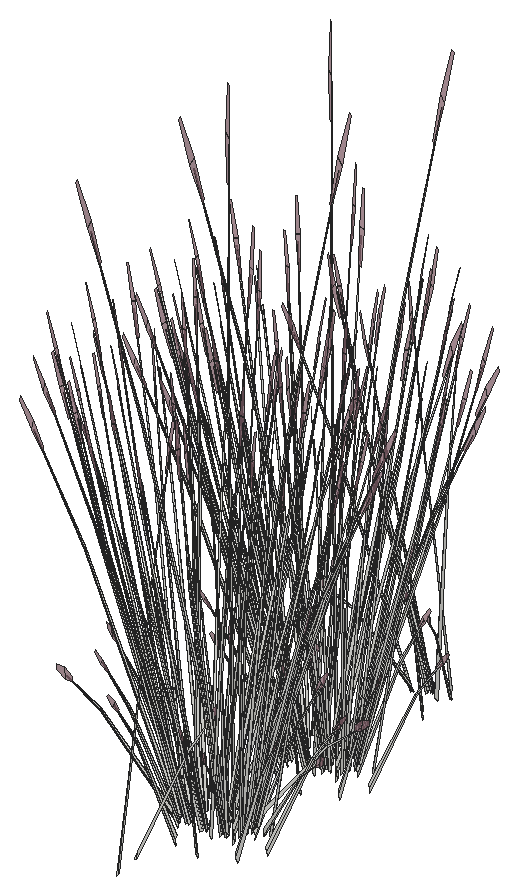
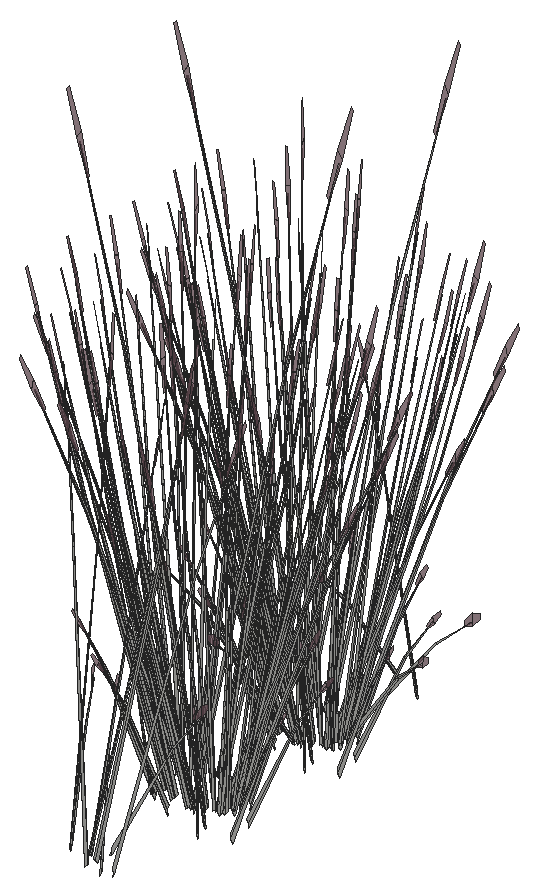
# SketchUp Ruby script. Lengths in inches.
U = 1.inch
M = Sketchup.active_model
def pt(a) = Geom::Point3d.new(a.map { |v| v * U })
def face(e, loops, mat)
  f = e.add_face(loops[0].map { |a| pt(a) })
  loops[1..].each { |l| e.add_face(l.map { |a| pt(a) }).erase! }
  f.material = f.back_material = mat if mat
  f
end
# faces: each face lists its corners as indices into pts; further lists are holes
def faces(e, pts, list, mat = nil) = list.each { |f| face(e, (f[0].is_a?(Array) ? f : [f]).map { |l| l.map { |i| pts[i] } }, mat) }
# xy, xz, yz: faces in a plane at the given z, y or x. An outline is a flat list of corners, or four numbers for a rectangle; further outlines are holes
def ring(l) = l.size == 4 ? [[l[0], l[1]], [l[2], l[1]], [l[2], l[3]], [l[0], l[3]]] : l.each_slice(2).to_a
def flat(e, list, mat, &to3) = list.each { |f| face(e, (f[0].is_a?(Array) ? f : [f]).map { |l| ring(l).map { |u, v| to3.(u, v) } }, mat) }
def xy(e, z, list, mat = nil) = flat(e, list, mat) { |x, y| [x, y, z] }
def xz(e, y, list, mat = nil) = flat(e, list, mat) { |x, z| [x, y, z] }
def yz(e, x, list, mat = nil) = flat(e, list, mat) { |y, z| [x, y, z] }
def lines(e, pts, list) = list.each { |a, b| e.add_line(pt(pts[a]), pt(pts[b])) }
# prism: a flat outline (further loops are holes) pulled along v
def prism(e, loops, v, mat = nil)
  f = face(e, loops, mat); d = Geom::Vector3d.new(v.map { |x| x * U })
  f.pushpull(f.normal.samedirection?(d) ? d.length : -d.length)
end
def box(e, o, s, mat = nil) = prism(e, [[o, [o[0] + s[0], o[1], o[2]], [o[0] + s[0], o[1] + s[1], o[2]], [o[0], o[1] + s[1], o[2]]]], [0, 0, s[2]], mat)
def at(x, y, z, deg = 0) = Geom::Transformation.translation(pt([x, y, z])) * Geom::Transformation.rotation(ORIGIN, Z_AXIS, deg.degrees)
def axes(o, x, y, z) = Geom::Transformation.new([*x, 0, *y, 0, *z, 0, *pt(o).to_a, 1])
def part(name) = M.definitions.add(name)
# library, detail: a bought-in or finely detailed component or shape, given as its bounding box
def library(name, o, s) = part(name).tap { |d| box(d.entities, o, s) }
def detail(e, o, s) = box(e.add_group.entities, o, s)
def put(e, d, t, mat = nil) = e.add_instance(d, t).tap { |i| i.material = mat if mat }
def group(e, t, mat = nil) = e.add_group.tap { |g| g.transformation = t; g.material = mat if mat }.entities
root = M.entities
M.materials.add("LightPink_Translucent").color = [144, 107, 117]
M.materials["LightPink_Translucent"].alpha = 0.75
c1 = part("blade")
p = [[2.15,0.21,22],[0,0.17,0],[0.09,0.45,0],[2.18,0.31,22],[2.29,0.31,22],[0.38,0.45,0],
  [2.48,0.24,33],[2.49,0.24,33],[2.48,0.22,33]]
faces(c1.entities,p,[[0,1,2,3],[4,5,2,3],[6,3,4,7],[8,0,3,6]])
c2 = part("seeds")
p = [[0.3,-0.1,1.38],[-0.01,-0.03,1.59],[-0.01,-0.03,0.03],[0.14,-0.07,-0.07],[0.29,-0.03,3],[0.15,0.01,3.11]]
faces(c2.entities,p,[[0,1,2,3],[1,0,4,5]],"LightPink_Translucent")
c3 = part("blade with seeds")
put(c3.entities,c1,at(0,0,0))
put(c3.entities,c2,axes([2.4,0.25,30.99],[1.5799,-0.05474,1.17369],[-0.12525,1.92788,0.29478],[-0.07173,-0.02425,1.56792]))
put(root,c3,axes([335.12,365.08,52.4],[0.01314,-0.36145,-0.62776],[0.55324,0.02428,0.07576],[0.05838,-0.15313,0.88802]))
put(root,c3,axes([333.14,359.24,52.17],[0.064,0.06292,1.54581],[0.51651,0.02472,-0.24447],[0.05194,0.13877,0.12397]))
put(root,c3,axes([335.89,364.51,52.17],[-0.00487,-0.07777,1.54581],[-0.41166,-0.22476,-0.24447],[0.06364,-0.13625,0.12397]))
put(root,c3,axes([334.16,364.5,52],[0.15222,-0.30049,-0.31292],[0.44409,0.08764,0.40398],[-0.04072,-0.12098,0.77298]))
put(root,c3,axes([334.5,364.9,51.43],[-0.09401,0.13431,1.51428],[-0.3944,-0.27795,0.12244],[0.17792,-0.17323,0.64734]))
put(root,c3,axes([333.93,364.7,52.14],[-0.49634,-0.09796,-0.45151],[0.17013,-0.33585,-0.34973],[-0.04551,-0.13522,0.86392]))
put(root,c3,axes([334.24,363.86,50.44],[0.06477,0.22786,1.01491],[-0.35932,-0.1262,0.74569],[0.03867,-0.11667,0.22354]))
put(root,c3,axes([335.01,364.96,52.14],[-0.36145,-0.26255,-0.45151],[0.38183,-0.22994,-0.34973],[0.055,-0.1334,0.86392]))
put(root,c3,axes([332.31,358.63,50.97],[0.01109,-0.20172,1.3638],[0.49896,0.10655,0.18846],[-0.04323,0.21498,0.64398]))
put(root,c3,axes([334.36,364.6875,52.45],[-0.49409,0.18193,-0.10745],[-0.24281,-0.32289,-0.59638],[-0.06519,-0.13607,0.90619]))
put(root,c3,axes([335.38,365.1,52.45],[-0.55492,-0.01936,-0.10745],[0.01517,-0.36657,-0.59638],[0.03855,-0.14118,0.90619]))
put(root,c3,axes([335.35,364.86,52],[0.34164,-0.20573,-0.31292],[0.3234,0.23491,0.40398],[0.04921,-0.11936,0.77298]))
put(root,c3,axes([332.39,364.14,50.44],[0.26338,0.136,1.01491],[-0.38358,0.08175,0.74569],[-0.08207,-0.10452,0.22354]))
put(root,c3,axes([333.03,364.86,52.4],[-0.43054,-0.18887,-0.62776],[0.30598,-0.33097,0.07576],[-0.15599,-0.11277,0.88802]))
put(root,c3,axes([332.88,364.61,52],[-0.07798,-0.31474,-0.31292],[0.44579,-0.08311,0.40398],[-0.11974,-0.09019,0.77298]))
put(root,c3,axes([331.92,365.07,51.43],[0.18755,0.06732,1.51428],[-0.38813,0.28243,0.12244],[-0.24191,-0.12741,0.64734]))
put(root,c3,axes([332.83,364.87,52.14],[-0.49824,0.09289,-0.45151],[-0.08716,-0.35177,-0.34973],[-0.13382,-0.10081,0.86392]))
put(root,c3,axes([335.77,365.71,52.4],[0.26374,-0.30832,-0.62776],[0.46217,0.21911,0.07576],[0.15748,-0.11171,0.88802]))
put(root,c3,axes([335.76,365.5625,52.14],[-0.12971,-0.3568,-0.45151],[0.49122,-0.06241,-0.34973],[0.14077,-0.09583,0.86392]))
put(root,c3,axes([331.88,364.45,52.17],[-0.10864,-0.00276,1.54581],[-0.34587,0.27582,-0.24447],[-0.18454,-0.05636,0.12397]))
put(root,c3,axes([335.99,365.82,52.45],[-0.46706,-0.21546,-0.10745],[0.26908,-0.31203,-0.59638],[0.13196,-0.10846,0.90619]))
put(root,c3,axes([334.06,367,50.9375],[0.43633,0.15757,1.33654],[-0.42745,0.33945,0.52853],[-0.19146,-0.20119,1.12046]))
put(root,c3,axes([336.36,364.85,50.44],[-0.16818,0.19891,1.01491],[-0.14456,-0.26725,0.74569],[0.1389,-0.06697,0.22354]))
put(root,c3,axes([336.12,365.6,52],[0.43951,-0.05584,-0.31292],[0.11606,0.31924,0.40398],[0.12595,-0.08575,0.77298]))
put(root,c3,axes([331.85,365.16,52],[-0.28729,-0.24465,-0.31292],[0.32804,-0.23159,0.40398],[-0.16667,-0.03524,0.77298]))
put(root,c3,axes([332.15,365.33,52.4],[-0.50473,-0.00941,-0.62776],[0.0339,-0.39618,0.07576],[-0.21383,-0.04181,0.88802]))
put(root,c3,axes([337.39,366.1,52.17],[0.07006,-0.05952,1.54581],[-0.08968,-0.3651,-0.24447],[0.1758,-0.06922,0.12397]))
put(root,c3,axes([331.98,365.41,52.14],[-0.36663,0.25884,-0.45151],[-0.32109,-0.27343,-0.34973],[-0.18628,-0.03938,0.86392]))
put(root,c3,axes([331.16,365.75,50.44],[0.32236,-0.02796,1.01491],[-0.20448,0.24636,0.74569],[-0.1593,-0.03696,0.22354]))
put(root,c3,axes([332.18,365.13,52.45],[-0.02704,0.39739,-0.10745],[-0.51189,-0.01086,-0.59638],[-0.19715,-0.0276,0.90619]))
put(root,c3,axes([336.01,366.66,52.45],[-0.25405,-0.35383,-0.10745],[0.45089,-0.17388,-0.59638],[0.19001,-0.04668,0.90619]))
put(root,c3,axes([335.98,366.36,52.14],[0.13679,-0.35544,-0.45151],[0.46898,0.12183,-0.34973],[0.18882,-0.03259,0.86392]))
put(root,c3,axes([331.52,365.68,51.43],[0.20943,-0.00885,1.51428],[-0.13893,0.38357,0.12244],[-0.29846,-0.02372,0.64734]))
put(root,c3,axes([335.9,366.49,52.4],[0.44368,-0.17257,-0.62776],[0.24726,0.35524,0.07576],[0.21437,-0.04035,0.88802]))
put(root,c3,axes([336.27,366.52,52],[0.41962,0.10901,-0.31292],[-0.12239,0.31802,0.40398],[0.16894,-0.02916,0.77298]))
put(root,c3,axes([331.34,366.01,52],[-0.41962,-0.10901,-0.31292],[0.12239,-0.31802,0.40398],[-0.16894,0.02916,0.77298]))
put(root,c3,axes([335.13,366.125,51.43],[-0.20943,0.00885,1.51428],[0.13893,-0.38357,0.12244],[0.29846,0.02372,0.64734]))
put(root,c3,axes([332.62,365.96,50.95],[0.14352,-0.05653,1.56454],[0.04949,0.39467,0.12244],[-0.31087,0.05237,0.55918]))
put(root,c3,axes([337.16,366.58,50.44],[-0.31197,0.06451,1.01491],[0.14684,-0.26661,0.74569],[0.1655,0.01824,0.22354]))
put(root,c3,axes([331.08,366.22,52.17],[-0.08245,0.05073,1.54581],[0.00701,0.37067,-0.24447],[-0.18899,0.0482,0.12397]))
put(root,c3,axes([331.63,366.17,52.14],[-0.13679,0.35544,-0.45151],[-0.46898,-0.12183,-0.34973],[-0.18882,0.03259,0.86392]))
put(root,c3,axes([331.61,365.87,52.45],[0.25405,0.35383,-0.10745],[-0.45089,0.17388,-0.59638],[-0.19001,0.04668,0.90619]))
put(root,c3,axes([336.62,367.4,51.47],[-0.09664,-0.32847,-0.03085],[0.45676,-0.07551,-0.13989],[0.09538,0.02082,0.4614]))
put(root,c3,axes([335.4375,367.39,52.45],[0.02704,-0.39739,-0.10745],[0.51189,0.01086,-0.59638],[0.19715,0.0276,0.90619]))
put(root,c3,axes([335.88,367.16,52.17],[0.10831,-0.00661,1.54581],[0.29709,-0.30358,-0.24447],[0.19266,0.04007,0.12397]))
put(root,c3,axes([331.61,366.36,51.43],[0.17519,-0.08265,1.51428],[0.14749,0.38193,0.12244],[-0.27504,0.08632,0.64734]))
put(root,c3,axes([335.46,367.2,52.4],[0.50473,0.00941,-0.62776],[-0.0339,0.39618,0.07576],[0.21383,0.04181,0.88802]))
put(root,c3,axes([330.7,367.69,50.44],[0.21042,-0.1771,1.01491],[0.08303,0.28036,0.74569],[-0.15207,0.0502,0.22354]))
put(root,c3,axes([335.77,367.37,52],[0.28729,0.24465,-0.31292],[-0.32804,0.23159,0.40398],[0.16667,0.03524,0.77298]))
put(root,c3,axes([331.49,366.93,52],[-0.43951,0.05584,-0.31292],[-0.11606,-0.31924,0.40398],[-0.12595,0.08575,0.77298]))
put(root,c3,axes([334.73,366.74,51.43],[-0.18755,-0.06732,1.51428],[0.38813,-0.28243,0.12244],[0.24191,0.12741,0.64734]))
put(root,c3,axes([334.77,365.85,51.95],[-0.4363,-0.20303,1.22187],[0.46069,-0.31611,0.5272],[0.14077,0.1905,1.18105]))
put(root,c3,axes([331.625,366.71,52.45],[0.46706,0.21546,-0.10745],[-0.26908,0.31203,-0.59638],[-0.13196,0.10846,0.90619]))
put(root,c3,axes([335.43,367.51,50.44],[-0.28429,-0.11236,1.01491],[0.36709,-0.11416,0.74569],[0.09901,0.0967,0.22354]))
put(root,c3,axes([334.43,367.83,52.45],[0.30087,-0.33447,-0.10745],[0.43572,0.19269,-0.59638],[0.15146,0.0945,0.90619]))
put(root,c3,axes([332.25,366.61,51.43],[0.12611,-0.12006,1.51428],[0.31843,0.32408,0.12244],[-0.2184,0.14759,0.64734]))
put(root,c3,axes([331.86,366.97,52.14],[0.12971,0.3568,-0.45151],[-0.49122,0.06241,-0.34973],[-0.14077,0.09583,0.86392]))
put(root,c3,axes([334.74,366.24,50.51],[-0.01379,-0.36791,1.24828],[0.62424,0.09537,0.52853],[-0.14764,0.20132,1.17828]))
put(root,c3,axes([334.79,367.66,52.14],[0.49824,-0.09289,-0.45151],[0.08716,0.35177,-0.34973],[0.13382,0.10081,0.86392]))
put(root,c3,axes([332.16,366.91,51.43],[0.09401,-0.13431,1.51428],[0.3944,0.27795,0.12244],[-0.17792,0.17323,0.64734]))
put(root,c3,axes([332.27,367.67,52],[-0.34164,0.20573,-0.31292],[-0.3234,-0.23491,0.40398],[-0.04921,0.11936,0.77298]))
put(root,c3,axes([331.09,367.61,52.17],[-0.01255,0.07733,1.54581],[0.35618,0.269,-0.24447],[-0.09325,0.12721,0.12397]))
put(root,c3,axes([333.25,367.84,52.45],[0.49409,-0.18193,-0.10745],[0.24281,0.32289,-0.59638],[0.06519,0.13607,0.90619]))
put(root,c3,axes([332.48,368.47,50.44],[-0.01307,-0.23234,1.01491],[0.32652,0.16572,0.74569],[-0.06422,0.11074,0.22354]))
put(root,c3,axes([332.61,367.57,52.42],[0.36145,0.26255,-0.50118],[-0.38183,0.22994,-0.3882],[-0.055,0.1334,0.95895]))
put(root,c3,axes([333.68,367.82,52.14],[0.49634,0.09796,-0.45151],[-0.17013,0.33585,-0.34973],[0.04551,0.13522,0.86392]))
put(root,c3,axes([333.96,367.13,51.43],[-0.11542,-0.12546,1.51428],[0.53333,-0.10562,0.12244],[0.12054,0.19696,0.64734]))
put(root,c3,axes([333.45,368.03,52],[-0.15222,0.30049,-0.31292],[-0.44409,-0.08764,0.40398],[0.04072,0.12098,0.77298]))
put(root,c3,axes([332.49,367.45,52.72],[-0.01314,0.36145,-0.69681],[-0.55324,-0.02428,0.08409],[-0.05838,0.15313,0.9857]))
put(root,c3,axes([332.69,374.15,51.43],[0.11542,0.12546,1.51428],[-0.53333,0.10562,0.12244],[-0.12054,-0.19696,0.64734]))
put(root,c3,axes([333.02,367.19,51.43],[-0.01236,-0.14998,1.51428],[0.53562,0.09949,0.12244],[-0.03313,0.21373,0.64734]))
put(root,c3,axes([334.11,374.24,52.4],[-0.24099,-0.31773,-0.62776],[0.49607,-0.17707,0.07576],[-0.05635,-0.15352,0.88802]))
put(root,c3,axes([333.5,367.76,52.4],[0.24099,0.31773,-0.62776],[-0.49607,0.17707,0.07576],[0.05635,0.15352,0.88802]))
put(root,c3,axes([333.14,368.5625,52.17],[0.064,0.06292,1.54581],[0.51651,0.02472,-0.24447],[0.05194,0.13877,0.12397]))
put(root,c3,axes([335.12,374.55,52.4],[0.01314,-0.36145,-0.62776],[0.55324,0.02428,0.07576],[0.05838,-0.15313,0.88802]))
put(root,c3,axes([334.16,373.97,52],[0.15222,-0.30049,-0.31292],[0.44409,0.08764,0.40398],[-0.04072,-0.12098,0.77298]))
put(root,c3,axes([334.5,374.37,51.43],[-0.09401,0.13431,1.51428],[-0.3944,-0.27795,0.12244],[0.17792,-0.17323,0.64734]))
put(root,c3,axes([333.93,374.18,52.14],[-0.49634,-0.09796,-0.45151],[0.17013,-0.33585,-0.34973],[-0.04551,-0.13522,0.86392]))
put(root,c3,axes([334.24,373.34,50.44],[0.06477,0.22786,1.01491],[-0.35932,-0.1262,0.74569],[0.03867,-0.11667,0.22354]))
put(root,c3,axes([332.31,367.96,50.97],[0.01109,-0.20172,1.3638],[0.49896,0.10655,0.18846],[-0.04323,0.21498,0.64398]))
put(root,c3,axes([335.01,374.43,52.14],[-0.36145,-0.26255,-0.45151],[0.38183,-0.22994,-0.34973],[0.055,-0.1334,0.86392]))
put(root,c3,axes([334.36,374.16,52.45],[-0.49409,0.18193,-0.10745],[-0.24281,-0.32289,-0.59638],[-0.06519,-0.13607,0.90619]))
put(root,c3,axes([335.38,374.57,52.45],[-0.55492,-0.01936,-0.10745],[0.01517,-0.36657,-0.59638],[0.03855,-0.14118,0.90619]))
put(root,c3,axes([335.35,374.33,52],[0.34164,-0.20573,-0.31292],[0.3234,0.23491,0.40398],[0.04921,-0.11936,0.77298]))
put(root,c3,axes([332.39,373.61,50.44],[0.26338,0.136,1.01491],[-0.38358,0.08175,0.74569],[-0.08207,-0.10452,0.22354]))
put(root,c3,axes([333.03,374.33,52.4],[-0.43054,-0.18887,-0.62776],[0.30598,-0.33097,0.07576],[-0.15599,-0.11277,0.88802]))
put(root,c3,axes([332.88,374.08,52],[-0.07798,-0.31474,-0.31292],[0.44579,-0.08311,0.40398],[-0.11974,-0.09019,0.77298]))
put(root,c3,axes([331.92,374.54,51.43],[0.18755,0.06732,1.51428],[-0.38813,0.28243,0.12244],[-0.24191,-0.12741,0.64734]))
put(root,c3,axes([332.83,374.34,52.14],[-0.49824,0.09289,-0.45151],[-0.08716,-0.35177,-0.34973],[-0.13382,-0.10081,0.86392]))
put(root,c3,axes([335.77,375.18,52.4],[0.26374,-0.30832,-0.62776],[0.46217,0.21911,0.07576],[0.15748,-0.11171,0.88802]))
put(root,c3,axes([335.76,375.04,52.14],[-0.12971,-0.3568,-0.45151],[0.49122,-0.06241,-0.34973],[0.14077,-0.09583,0.86392]))
put(root,c3,axes([335.99,375.29,52.45],[-0.46706,-0.21546,-0.10745],[0.26908,-0.31203,-0.59638],[0.13196,-0.10846,0.90619]))
put(root,c3,axes([334.06,376.47,50.9375],[0.43633,0.15757,1.33654],[-0.42745,0.33945,0.52853],[-0.19146,-0.20119,1.12046]))
put(root,c3,axes([336.36,374.33,50.44],[-0.16818,0.19891,1.01491],[-0.14456,-0.26725,0.74569],[0.1389,-0.06697,0.22354]))
put(root,c3,axes([336.12,375.07,52],[0.43951,-0.05584,-0.31292],[0.11606,0.31924,0.40398],[0.12595,-0.08575,0.77298]))
put(root,c3,axes([331.85,374.63,52],[-0.28729,-0.24465,-0.31292],[0.32804,-0.23159,0.40398],[-0.16667,-0.03524,0.77298]))
put(root,c3,axes([332.15,374.8,52.4],[-0.50473,-0.00941,-0.62776],[0.0339,-0.39618,0.07576],[-0.21383,-0.04181,0.88802]))
put(root,c3,axes([331.98,374.88,52.14],[-0.36663,0.25884,-0.45151],[-0.32109,-0.27343,-0.34973],[-0.18628,-0.03938,0.86392]))
put(root,c3,axes([331.16,375.22,50.44],[0.32236,-0.02796,1.01491],[-0.20448,0.24636,0.74569],[-0.1593,-0.03696,0.22354]))
put(root,c3,axes([332.18,374.61,52.45],[-0.02704,0.39739,-0.10745],[-0.51189,-0.01086,-0.59638],[-0.19715,-0.0276,0.90619]))
put(root,c3,axes([336.01,376.13,52.45],[-0.25405,-0.35383,-0.10745],[0.45089,-0.17388,-0.59638],[0.19001,-0.04668,0.90619]))
put(root,c3,axes([335.98,375.83,52.14],[0.13679,-0.35544,-0.45151],[0.46898,0.12183,-0.34973],[0.18882,-0.03259,0.86392]))
put(root,c3,axes([331.52,375.15,51.43],[0.20943,-0.00885,1.51428],[-0.13893,0.38357,0.12244],[-0.29846,-0.02372,0.64734]))
put(root,c3,axes([335.9,375.96,52.4],[0.44368,-0.17257,-0.62776],[0.24726,0.35524,0.07576],[0.21437,-0.04035,0.88802]))
put(root,c3,axes([336.27,375.99,52],[0.41962,0.10901,-0.31292],[-0.12239,0.31802,0.40398],[0.16894,-0.02916,0.77298]))
put(root,c3,axes([331.34,375.48,52],[-0.41962,-0.10901,-0.31292],[0.12239,-0.31802,0.40398],[-0.16894,0.02916,0.77298]))
put(root,c3,axes([335.13,375.6,51.43],[-0.20943,0.00885,1.51428],[0.13893,-0.38357,0.12244],[0.29846,0.02372,0.64734]))
put(root,c3,axes([332.62,375.43,50.95],[0.14352,-0.05653,1.56454],[0.04949,0.39467,0.12244],[-0.31087,0.05237,0.55918]))
put(root,c3,axes([337.16,376.05,50.44],[-0.31197,0.06451,1.01491],[0.14684,-0.26661,0.74569],[0.1655,0.01824,0.22354]))
put(root,c3,axes([331.63,375.65,52.14],[-0.13679,0.35544,-0.45151],[-0.46898,-0.12183,-0.34973],[-0.18882,0.03259,0.86392]))
put(root,c3,axes([331.61,375.34,52.45],[0.25405,0.35383,-0.10745],[-0.45089,0.17388,-0.59638],[-0.19001,0.04668,0.90619]))
put(root,c3,axes([336.62,376.875,51.47],[-0.09664,-0.32847,-0.03085],[0.45676,-0.07551,-0.13989],[0.09538,0.02082,0.4614]))
put(root,c3,axes([335.4375,376.87,52.45],[0.02704,-0.39739,-0.10745],[0.51189,0.01086,-0.59638],[0.19715,0.0276,0.90619]))
put(root,c3,axes([331.61,375.83,51.43],[0.17519,-0.08265,1.51428],[0.14749,0.38193,0.12244],[-0.27504,0.08632,0.64734]))
put(root,c3,axes([335.46,376.68,52.4],[0.50473,0.00941,-0.62776],[-0.0339,0.39618,0.07576],[0.21383,0.04181,0.88802]))
put(root,c3,axes([330.7,377.17,50.44],[0.21042,-0.1771,1.01491],[0.08303,0.28036,0.74569],[-0.15207,0.0502,0.22354]))
put(root,c3,axes([335.77,376.84,52],[0.28729,0.24465,-0.31292],[-0.32804,0.23159,0.40398],[0.16667,0.03524,0.77298]))
put(root,c3,axes([331.49,376.4,52],[-0.43951,0.05584,-0.31292],[-0.11606,-0.31924,0.40398],[-0.12595,0.08575,0.77298]))
put(root,c3,axes([334.73,376.21,51.43],[-0.18755,-0.06732,1.51428],[0.38813,-0.28243,0.12244],[0.24191,0.12741,0.64734]))
put(root,c3,axes([334.77,375.33,51.95],[-0.4363,-0.20303,1.22187],[0.46069,-0.31611,0.5272],[0.14077,0.1905,1.18105]))
put(root,c3,axes([331.625,376.18,52.45],[0.46706,0.21546,-0.10745],[-0.26908,0.31203,-0.59638],[-0.13196,0.10846,0.90619]))
put(root,c3,axes([335.43,376.98,50.44],[-0.28429,-0.11236,1.01491],[0.36709,-0.11416,0.74569],[0.09901,0.0967,0.22354]))
put(root,c3,axes([334.43,377.3,52.45],[0.30087,-0.33447,-0.10745],[0.43572,0.19269,-0.59638],[0.15146,0.0945,0.90619]))
put(root,c3,axes([332.25,376.09,51.43],[0.12611,-0.12006,1.51428],[0.31843,0.32408,0.12244],[-0.2184,0.14759,0.64734]))
put(root,c3,axes([331.86,376.4375,52.14],[0.12971,0.3568,-0.45151],[-0.49122,0.06241,-0.34973],[-0.14077,0.09583,0.86392]))
put(root,c3,axes([334.74,375.71,50.51],[-0.01379,-0.36791,1.24828],[0.62424,0.09537,0.52853],[-0.14764,0.20132,1.17828]))
put(root,c3,axes([334.79,377.13,52.14],[0.49824,-0.09289,-0.45151],[0.08716,0.35177,-0.34973],[0.13382,0.10081,0.86392]))
put(root,c3,axes([332.16,376.38,51.43],[0.09401,-0.13431,1.51428],[0.3944,0.27795,0.12244],[-0.17792,0.17323,0.64734]))
put(root,c3,axes([332.27,377.14,52],[-0.34164,0.20573,-0.31292],[-0.3234,-0.23491,0.40398],[-0.04921,0.11936,0.77298]))
put(root,c3,axes([333.25,377.3125,52.45],[0.49409,-0.18193,-0.10745],[0.24281,0.32289,-0.59638],[0.06519,0.13607,0.90619]))
put(root,c3,axes([332.48,377.9375,50.44],[-0.01307,-0.23234,1.01491],[0.32652,0.16572,0.74569],[-0.06422,0.11074,0.22354]))
put(root,c3,axes([332.61,377.04,52.42],[0.36145,0.26255,-0.50118],[-0.38183,0.22994,-0.3882],[-0.055,0.1334,0.95895]))
put(root,c3,axes([333.68,377.3,52.14],[0.49634,0.09796,-0.45151],[-0.17013,0.33585,-0.34973],[0.04551,0.13522,0.86392]))
put(root,c3,axes([333.96,376.6,51.43],[-0.11542,-0.12546,1.51428],[0.53333,-0.10562,0.12244],[0.12054,0.19696,0.64734]))
put(root,c3,axes([333.45,377.5,52],[-0.15222,0.30049,-0.31292],[-0.44409,-0.08764,0.40398],[0.04072,0.12098,0.77298]))
put(root,c3,axes([332.49,376.92,52.72],[-0.01314,0.36145,-0.69681],[-0.55324,-0.02428,0.08409],[-0.05838,0.15313,0.9857]))
put(root,c3,axes([333.02,376.67,51.43],[-0.01236,-0.14998,1.51428],[0.53562,0.09949,0.12244],[-0.03313,0.21373,0.64734]))
put(root,c3,axes([333.5,377.23,52.4],[0.24099,0.31773,-0.62776],[-0.49607,0.17707,0.07576],[0.05635,0.15352,0.88802]))
put(root,c3,axes([332.31,377.43,50.97],[0.01109,-0.20172,1.3638],[0.49896,0.10655,0.18846],[-0.04323,0.21498,0.64398]))
put(root,c3,axes([332.69,385.46,51.43],[0.11542,0.12546,1.51428],[-0.53333,0.10562,0.12244],[-0.12054,-0.19696,0.64734]))
put(root,c3,axes([333.57,384.625,52.17],[-0.07723,-0.05479,1.54581],[-0.51538,0.03473,-0.24447],[-0.08225,-0.13104,0.12397]))
put(root,c3,axes([334.11,385.55,52.4],[-0.24099,-0.31773,-0.62776],[0.49607,-0.17707,0.07576],[-0.05635,-0.15352,0.88802]))
put(root,c3,axes([335.12,385.86,52.4],[0.01314,-0.36145,-0.62776],[0.55324,0.02428,0.07576],[0.05838,-0.15313,0.88802]))
put(root,c3,axes([335.89,385.3,52.17],[-0.00487,-0.07777,1.54581],[-0.41166,-0.22476,-0.24447],[0.06364,-0.13625,0.12397]))
put(root,c3,axes([334.16,385.28,52],[0.15222,-0.30049,-0.31292],[0.44409,0.08764,0.40398],[-0.04072,-0.12098,0.77298]))
put(root,c3,axes([334.5,385.68,51.43],[-0.09401,0.13431,1.51428],[-0.3944,-0.27795,0.12244],[0.17792,-0.17323,0.64734]))
put(root,c3,axes([333.93,385.49,52.14],[-0.49634,-0.09796,-0.45151],[0.17013,-0.33585,-0.34973],[-0.04551,-0.13522,0.86392]))
put(root,c3,axes([334.24,384.64,50.44],[0.06477,0.22786,1.01491],[-0.35932,-0.1262,0.74569],[0.03867,-0.11667,0.22354]))
